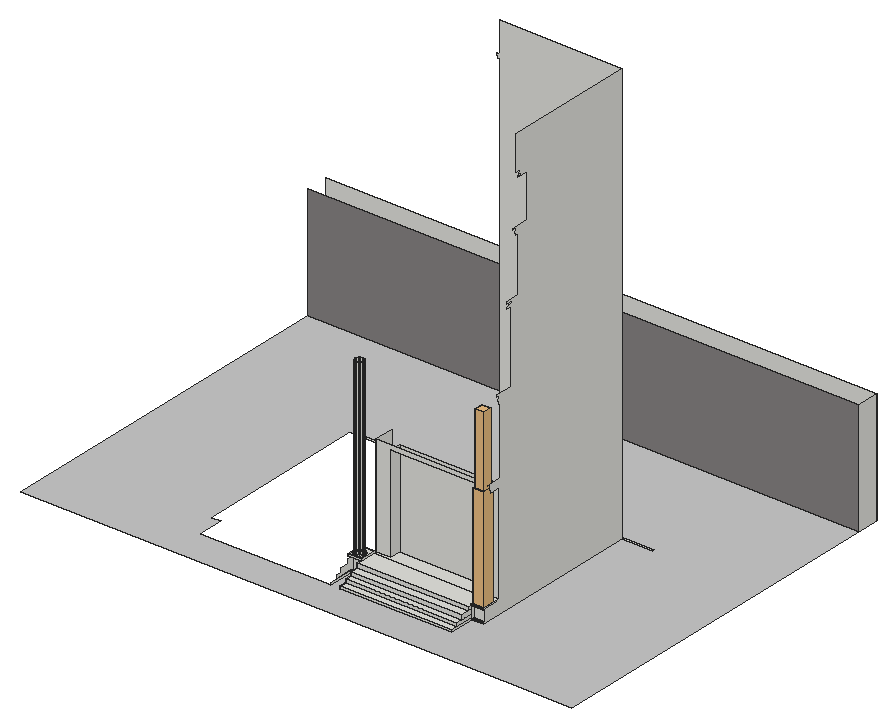
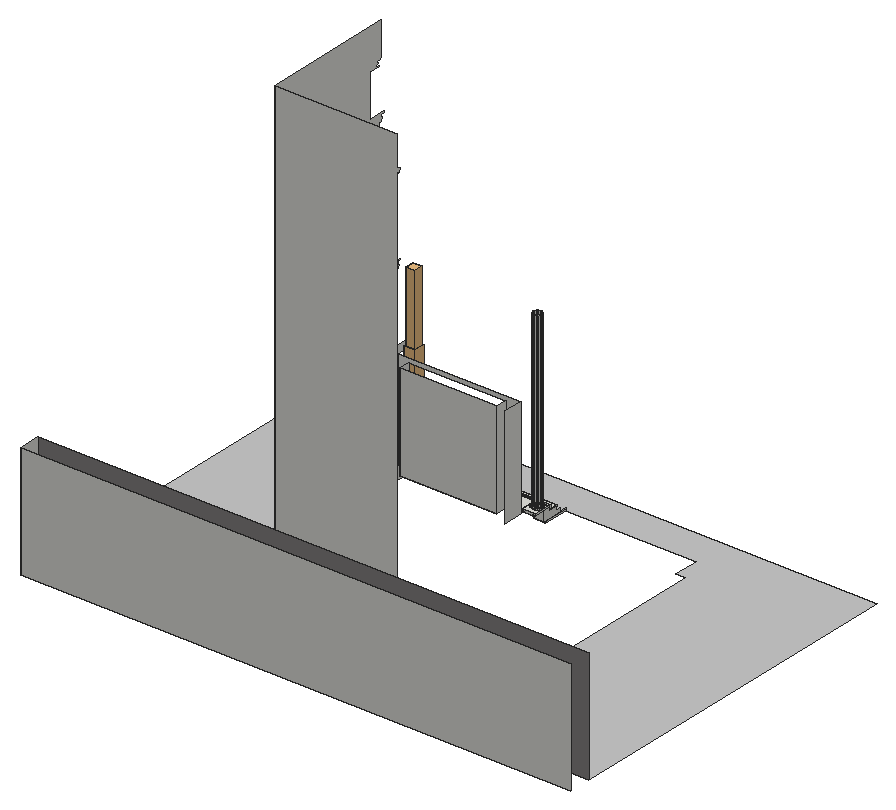
# SketchUp Ruby script. Lengths in inches.
U = 1.inch
M = Sketchup.active_model
def pt(a) = Geom::Point3d.new(a.map { |v| v * U })
def face(e, loops, mat)
  f = e.add_face(loops[0].map { |a| pt(a) })
  loops[1..].each { |l| e.add_face(l.map { |a| pt(a) }).erase! }
  f.material = f.back_material = mat if mat
  f
end
# faces: each face lists its corners as indices into pts; further lists are holes
def faces(e, pts, list, mat = nil) = list.each { |f| face(e, (f[0].is_a?(Array) ? f : [f]).map { |l| l.map { |i| pts[i] } }, mat) }
# xy, xz, yz: faces in a plane at the given z, y or x. An outline is a flat list of corners, or four numbers for a rectangle; further outlines are holes
def ring(l) = l.size == 4 ? [[l[0], l[1]], [l[2], l[1]], [l[2], l[3]], [l[0], l[3]]] : l.each_slice(2).to_a
def flat(e, list, mat, &to3) = list.each { |f| face(e, (f[0].is_a?(Array) ? f : [f]).map { |l| ring(l).map { |u, v| to3.(u, v) } }, mat) }
def xy(e, z, list, mat = nil) = flat(e, list, mat) { |x, y| [x, y, z] }
def xz(e, y, list, mat = nil) = flat(e, list, mat) { |x, z| [x, y, z] }
def yz(e, x, list, mat = nil) = flat(e, list, mat) { |y, z| [x, y, z] }
def lines(e, pts, list) = list.each { |a, b| e.add_line(pt(pts[a]), pt(pts[b])) }
# prism: a flat outline (further loops are holes) pulled along v
def prism(e, loops, v, mat = nil)
  f = face(e, loops, mat); d = Geom::Vector3d.new(v.map { |x| x * U })
  f.pushpull(f.normal.samedirection?(d) ? d.length : -d.length)
end
def box(e, o, s, mat = nil) = prism(e, [[o, [o[0] + s[0], o[1], o[2]], [o[0] + s[0], o[1] + s[1], o[2]], [o[0], o[1] + s[1], o[2]]]], [0, 0, s[2]], mat)
def at(x, y, z, deg = 0) = Geom::Transformation.translation(pt([x, y, z])) * Geom::Transformation.rotation(ORIGIN, Z_AXIS, deg.degrees)
def axes(o, x, y, z) = Geom::Transformation.new([*x, 0, *y, 0, *z, 0, *pt(o).to_a, 1])
def part(name) = M.definitions.add(name)
# library, detail: a bought-in or finely detailed component or shape, given as its bounding box
def library(name, o, s) = part(name).tap { |d| box(d.entities, o, s) }
def detail(e, o, s) = box(e.add_group.entities, o, s)
def put(e, d, t, mat = nil) = e.add_instance(d, t).tap { |i| i.material = mat if mat }
def group(e, t, mat = nil) = e.add_group.tap { |g| g.transformation = t; g.material = mat if mat }.entities
root = M.entities
M.materials.add("[Brick Tumbled]").color = [135, 132, 132]
M.materials.add("[Cladding Stucco White]").color = [200, 200, 200]
c1 = library("Group\#1",[0,0,0],[8.125,8.125,76.3125])
xy(root,0,[[107.37,172.5625,326.68,174.07],[326.68,264.36,404.87,280.51]])
xy(root,0,[[0,0,355.49,0,355.49,0.34,404.87,0.34,404.87,264.36,326.68,264.36,326.68,172.5625,304.48,172.5625,304.48,44.88,295.89,44.88,295.89,26.25,214.17,26.25,214.17,44.88,207.4,44.88,207.4,26.25,111.24,26.25,111.24,44.88,104.23,44.88,104.23,172.5625,107.37,172.5625,107.37,174.07,326.68,174.07,326.68,264.36,0,264.36]],"[Cladding Stucco White]")
xy(root,0.71,[[296.3,44.88,304.48,45.25]])
xy(root,0.92,[[296.3,45.25,304.48,46.63]])
xy(root,1.01,[[207.37,26.25,207.4,44.88],[207.4,44.88,214.17,45.32]])
xy(root,1.55,[[207.37,45.32,214.17,46.63]])
xy(root,3.94,[[214.17,31.63,295.89,35.75]])
xy(root,6.875,[[214.17,35.75,295.89,41.88]])
xy(root,9.8125,[[214.17,41.88,295.89,41.88,295.89,56.16,214.17,56.57],[295.89,44.44,295.89,44.88,296.3,44.88,296.3,46.63,304.48,46.63,304.48,44.88,304.66,44.88,304.66,44.44],[304.48,44.88,304.66,56.12],[295.89,56.16,296.02,56.16,296.02,57.2,296.52,57.2,296.52,67.33,225.14,67.33,225.14,59.39,214.17,59.39,214.17,56.57]])
xy(root,10.4375,[[[295.89,44.44,304.66,44.44,304.66,56.12,304.48,56.12,304.48,59.39,296.52,59.39,296.52,57.2,296.02,57.2,296.02,56.16,295.89,56.16],[300.02,45.77,298.97,45.93,298,46.36,297.17,47.02,296.54,47.87,296.15,48.86,296.03,49.91,296.19,50.96,296.62,51.93,297.28,52.76,298.13,53.39,299.12,53.78,300.18,53.9,301.22,53.74,302.2,53.3125,303.02,52.65,303.65,51.8,304.04,50.81,304.16,49.75,304,48.71,303.57,47.73,302.91,46.91,302.06,46.28,301.07,45.89]]])
xy(root,10.75,[[205.39,44.25,205.39,44.88,206.95,44.88,206.95,46.44,207.18,46.125,208.01,45.46,208.98,45.04,210.03,44.88,211.08,45,212.07,45.38,212.93,46.01,213.42,46.63,214.17,46.63,214.17,44.88,215.3,44.88,215.3,44.25],[205.39,44.88,205.39,47.4,206.39,47.4,206.55,46.98,206.95,46.44,206.95,44.88],[210.03,44.88,208.98,45.04,208.01,45.46,207.18,46.125,206.95,46.44,206.95,46.63,210.03,46.63],[210.03,44.88,210.03,46.63,213.42,46.63,212.93,46.01,212.07,45.38,211.08,45],[214.17,44.88,215.3,56.57],
  [206.95,46.44,206.55,46.98,206.39,47.4,205.39,47.4,205.39,50.48,206.39,50.48,206.63,51.04,206.95,51.4375],[205.39,50.48,205.39,56.57,206.95,56.57,206.95,51.4375,206.63,51.04,206.39,50.48]])
xy(root,11.6875,[[205.39,44.25,215.3,56.57]])
xy(root,12,[[[210.03,44.88,211.08,45,212.07,45.38,212.93,46.01,213.59,46.84,214.01,47.8125,214.17,48.86,214.05,49.91,213.67,50.9,213.04,51.76,212.21,52.42,211.24,52.84,210.19,53,209.14,52.89,208.15,52.5,207.29,51.87,206.63,51.04,206.21,50.07,206.05,49.02,206.17,47.97,206.55,46.98,207.18,46.125,208.01,45.46,208.98,45.04],[210.04,45.32,209.1,45.46,208.23,45.84,207.5,46.43,206.93,47.19,206.59,48.07,206.48,49.01,206.625,49.95,207.01,50.82,207.6,51.56,208.36,52.12,209.24,52.46,210.18,52.57,211.12,52.43,211.98,52.05,212.72,51.45,213.29,50.69,213.63,49.81,213.74,48.87,213.59,47.93,213.21,47.07,212.62,46.33,211.86,45.77,210.98,45.42]]])
xy(root,12.875,[[[210.04,45.32,210.98,45.42,211.86,45.77,212.62,46.33,213.21,47.07,213.59,47.93,213.74,48.87,213.63,49.81,213.29,50.69,212.72,51.45,211.98,52.05,211.12,52.43,210.18,52.57,209.24,52.46,208.36,52.12,207.6,51.56,207.01,50.82,206.625,49.95,206.48,49.01,206.59,48.07,206.93,47.19,207.5,46.43,208.23,45.84,209.1,45.46],[210.05,45.88,209.26,46,208.53,46.32,207.9,46.82,207.43,47.46,207.14,48.21,207.05,49,207.17,49.79,207.49,50.52,207.99,51.15,208.63,51.625,209.375,51.91,210.17,52,210.96,51.88,211.69,51.5625,212.32,51.0625,212.79,50.42,213.08,49.68,213.17,48.88,213.05,48.09,212.73,47.36,212.23,46.73,211.59,46.26,210.84,45.97]]])
xy(root,15.4375,[[[210.09,45.77,210.9,45.86,211.66,46.15,212.32,46.63,212.83,47.27,213.15,48.02,213.28,48.83,213.1875,49.64,212.89,50.4,212.41,51.06,211.77,51.57,211.02,51.89,210.22,52.02,209.41,51.93,208.65,51.63,207.99,51.15,207.48,50.51,207.15,49.77,207.03,48.96,207.11,48.15,207.41,47.39,207.89,46.73,208.53,46.22,209.28,45.89],[210.05,46.14,209.33,46.25,208.66,46.55,208.09,47,207.66,47.59,207.39,48.27,207.3125,49,207.42,49.72,207.72,50.39,208.17,50.96,208.76,51.39,209.44,51.66,210.17,51.74,210.89,51.63,211.56,51.34,212.125,50.88,212.56,50.29,212.83,49.61,212.91,48.89,212.8,48.16,212.5,47.5,212.05,46.92,211.46,46.49,210.78,46.23]]])
xy(root,15.5625,[[[210.05,45.68,210.89,45.77,211.6875,46.08,212.37,46.59,212.9,47.25,213.25,48.03,213.375,48.875,213.28,49.72,212.97,50.52,212.46,51.2,211.8,51.74,211.02,52.08,210.17,52.21,209.33,52.11,208.53,51.8,207.85,51.3,207.32,50.63,206.97,49.85,206.85,49.01,206.94,48.16,207.25,47.37,207.76,46.68,208.42,46.15,209.2,45.81],[210.09,45.77,209.28,45.89,208.53,46.22,207.89,46.73,207.41,47.39,207.11,48.15,207.03,48.96,207.15,49.77,207.48,50.51,207.99,51.15,208.65,51.63,209.41,51.93,210.22,52.02,211.02,51.89,211.77,51.57,212.41,51.06,212.89,50.4,213.1875,49.64,213.28,48.83,213.15,48.02,212.83,47.27,212.32,46.63,211.66,46.15,210.9,45.86]]])
xz(root,26.25,[[214.17,0,295.89,0,295.89,1.36,214.17,1.55]])
xz(root,31.63,[[295.89,1.36,295.89,3.94,214.17,3.94,214.17,1.55]])
xz(root,35.75,[[214.17,3.94,295.89,6.875]])
xz(root,41.88,[[214.17,6.875,295.89,9.8125]])
xz(root,44.25,[[205.39,10.75,215.3,11.6875]])
xz(root,44.44,[[295.89,9.8125,304.66,10.4375]])
xz(root,44.88,[[207.4,0,207.45,0,207.4,1.01],[207.45,0,214.17,0,214.17,1.01,207.4,1.01],[295.89,0,296.3,0,296.3,1.35,295.89,1.36],[296.3,0,304.48,0.71],[207.37,1.01,207.4,1.01,207.37,1.55],
  [296.3,1.35,296.3,9.8125,295.89,9.8125,295.89,1.36]])
xz(root,45.25,[[296.3,0.71,304.48,0.92]])
xz(root,45.32,[[207.4,1.01,214.17,1.01,214.17,1.55,207.37,1.55]])
xz(root,46.63,[[296.3,0.92,304.48,9.8125],[207.37,1.55,214.17,1.55,214.17,10.75,206.95,10.75,206.95,9.8125]])
xz(root,56.12,[[304.48,9.8125,304.66,10.4375]])
xz(root,56.16,[[295.89,9.8125,296.02,10.4375]])
xz(root,56.57,[[206.95,9.8125,206.95,10.75,205.39,10.75,205.39,11.6875,215.3,11.6875,215.3,10.75,214.17,10.75,214.17,9.8125]])
xz(root,57.2,[[296.02,9.8125,296.52,10.4375]])
xz(root,59.39,[[214.17,9.8125,225.14,9.8125,225.14,80.55,296.52,80.55,296.52,10.4375,304.48,10.4375,304.48,83.64,214.17,83.64]])
xz(root,67.33,[[225.14,9.8125,296.52,80.55]])
xz(root,172.5625,[[214.17,0,214.17,284.98,212.73,284.98,212.73,286.66,212.55,286.66,212.55,288.01,214.17,288.01,214.17,309.9375,304.48,309.9375,304.48,0]])
xz(root,264.36,[[0,0,404.87,83.4375]],"[Brick Tumbled]")
xz(root,280.51,[[0,0,404.87,83.4375]])
yz(root,205.39,[[44.25,10.75,56.57,11.6875]])
yz(root,206.95,[[46.63,9.8125,56.57,10.75]])
yz(root,207.37,[[26.25,1.01,44.88,1.55]])
yz(root,207.4,[[26.25,0,44.88,1.01]])
yz(root,214.17,[[26.25,0,44.88,1.01],[26.25,1.01,45.32,1.55],[31.63,1.55,31.63,3.94,35.75,3.94,35.75,6.875,41.88,6.875,41.88,9.8125,46.63,9.8125,46.63,1.55],[46.63,9.8125,56.57,10.75],[59.39,9.8125,73.64,83.92]])
yz(root,215.3,[[44.25,10.75,56.57,11.6875]])
yz(root,225.14,[[59.39,9.8125,67.33,80.55]])
yz(root,295.89,[[26.25,0,44.88,1.36],[31.63,1.36,44.88,3.94],[35.75,3.94,44.88,6.875],[41.88,6.875,44.88,9.8125],[44.44,9.8125,56.16,10.4375]])
yz(root,296.02,[[56.16,9.8125,57.2,10.4375]])
yz(root,296.3,[[44.88,0.71,45.25,1.35],[45.25,0.92,46.63,0.92,46.63,9.8125,44.88,9.8125,44.88,1.35,45.25,1.35]])
yz(root,296.52,[[57.2,9.8125,57.2,10.4375,59.39,10.4375,59.39,80.55,67.33,80.55,67.33,9.8125]])
yz(root,304.48,[[44.88,0,172.5625,0,172.5625,309.9375,74.52,309.9375,74.52,284.98,75.52,284.98,75.52,284.33,78.58,284.33,78.58,282.84,77.08,282.84,77.08,282.12,79.14,282.12,79.14,281.14,76.7,281.14,76.7,280.4,85.02,280.4,85.02,248.6875,71.75,248.6875,71.75,247.95,74.625,247.95,74.625,245.88,73.625,245.88,73.625,244.86,74.375,244.86,74.375,243.8,75.125,243.8,75.125,243.18,76.3125,243.18,76.3125,202.875,66.1875,202.875,66.1875,201.42,71,201.42,71,199.99,68.5625,199.99,68.5625,199.04,66.56,199.04,66.56,197.93,70.1875,197.93,70.1875,145.3125,57.25,145.3125,57.25,144.42,59.19,144.42,59.19,141.75,58,141.75,58,141.14,59.06,141.14,59.06,139.125,60.44,139.125,60.44,89.5625,49.08,89.5625,49.08,89.28,50.51,89.28,50.51,86.32,51.58,86.32,51.58,83.64,59.39,83.64,59.39,10.4375,56.12,10.4375,56.12,9.8125,46.63,9.8125,46.63,0.92,45.25,0.92,45.25,0.71,44.88,0.71]])
yz(root,304.66,[[44.44,9.8125,56.12,10.4375]])
yz(root,404.87,[[264.36,0,280.51,83.4375]])
p = [[207.37,44.88,1.55],[207.4,44.88,1.01],[207.4,45.32,1.01],[207.37,45.32,1.55],[295.89,26.25,1.36],[295.89,31.63,1.36],
  [214.17,31.63,1.55],[214.17,26.25,1.55],[206.95,46.63,9.8125],[206.95,41.88,9.8125],[207.1,41.88,6.88],[207.1,35.75,6.88],
  [207.25,35.75,3.95],[207.25,31.63,3.95],[207.37,31.63,1.55],[207.37,46.63,1.55],[213.42,46.63,10.75],[213.59,46.84,10.75],
  [213.59,46.84,12],[212.93,46.01,12],[212.93,46.01,10.75],[206.95,46.44,10.75],[207.18,46.125,10.75],[207.18,46.125,12],
  [206.55,46.98,12],[206.55,46.98,10.75],[214.01,47.8125,10.75],[214.01,47.8125,12],[206.39,47.4,10.75],[206.17,47.97,12],
  [206.17,47.97,10.75],[214.17,48.86,10.75],[214.17,48.86,12],[206.05,49.02,10.75],[206.05,49.02,12],[214.05,49.91,10.75],
  [214.05,49.91,12],[206.21,50.07,10.75],[206.21,50.07,12],[213.67,50.9,10.75],[213.67,50.9,12],[206.39,50.48,10.75],
  [206.63,51.04,12],[206.63,51.04,10.75],[213.04,51.76,10.75],[213.04,51.76,12],[206.95,51.4375,10.75],[207.29,51.87,12],
  [207.29,51.87,10.75],[212.21,52.42,10.75],[212.21,52.42,12],[208.15,52.5,10.75],[208.15,52.5,12],[211.24,52.84,10.75],
  [211.24,52.84,12],[209.14,52.89,10.75],[209.14,52.89,12],[210.19,53,10.75],[210.19,53,12],[208.98,45.04,10.75],
  [210.03,44.88,10.75],[210.03,44.88,12],[208.98,45.04,12],[211.08,45,10.75],[211.08,45,12],[208.01,45.46,10.75],
  [208.01,45.46,12],[212.07,45.38,10.75],[212.07,45.38,12],[209.1,45.46,12],[210.04,45.32,12],[210.04,45.32,12.875],
  [209.1,45.46,12.875],[210.98,45.42,12],[210.98,45.42,12.875],[211.86,45.77,12],[211.86,45.77,12.875],[208.23,45.84,12],
  [208.23,45.84,12.875],[207.5,46.43,12],[207.5,46.43,12.875],[212.62,46.33,12],[212.62,46.33,12.875],[213.21,47.07,12],
  [213.21,47.07,12.875],[206.93,47.19,12],[206.93,47.19,12.875],[213.59,47.93,12],[213.59,47.93,12.875],[206.59,48.07,12],
  [206.59,48.07,12.875],[213.74,48.87,12],[213.74,48.87,12.875],[206.48,49.01,12],[206.48,49.01,12.875],[213.63,49.81,12],
  [213.63,49.81,12.875],[206.625,49.95,12],[206.625,49.95,12.875],[213.29,50.69,12],[213.29,50.69,12.875],[207.01,50.82,12],
  [207.01,50.82,12.875],[212.72,51.45,12],[212.72,51.45,12.875],[207.6,51.56,12],[207.6,51.56,12.875],[211.98,52.05,12],
  [211.98,52.05,12.875],[208.36,52.12,12],[208.36,52.12,12.875],[211.12,52.43,12],[211.12,52.43,12.875],[209.24,52.46,12],
  [209.24,52.46,12.875],[210.18,52.57,12],[210.18,52.57,12.875],[210.05,45.88,139.125],[209.26,46,139.125],[209.26,46,12.875],
  [210.05,45.88,12.875],[210.84,45.97,139.125],[210.84,45.97,12.875],[208.53,46.32,139.125],[208.53,46.32,12.875],[211.59,46.26,139.125],
  [211.59,46.26,12.875],[207.9,46.82,139.125],[207.9,46.82,12.875],[212.23,46.73,139.125],[212.23,46.73,12.875],[212.73,47.36,139.125],
  [212.73,47.36,12.875],[207.43,47.46,139.125],[207.43,47.46,12.875],[213.05,48.09,139.125],[213.05,48.09,12.875],[207.14,48.21,139.125],
  [207.14,48.21,12.875],[213.17,48.88,139.125],[213.17,48.88,12.875],[207.05,49,139.125],[207.05,49,12.875],[213.08,49.68,139.125],
  [213.08,49.68,12.875],[207.17,49.79,139.125],[207.17,49.79,12.875],[212.79,50.42,139.125],[212.79,50.42,12.875],[207.49,50.52,139.125],
  [207.49,50.52,12.875],[212.32,51.0625,139.125],[212.32,51.0625,12.875],[207.99,51.15,139.125],[207.99,51.15,15.5625],[207.99,51.15,15.4375],
  [207.99,51.15,14.6875],[207.99,51.15,12.875],[208.63,51.625,139.125],[208.63,51.625,12.875],[211.69,51.5625,139.125],[211.69,51.5625,12.875],
  [209.375,51.91,139.125],[209.375,51.91,12.875],[210.96,51.88,139.125],[210.96,51.88,12.875],[210.17,52,139.125],[210.17,52,12.875],
  [209.28,45.89,14.6875],[210.09,45.77,14.6875],[210.09,45.77,15.4375],[209.28,45.89,15.4375],[210.9,45.86,14.6875],[210.9,45.86,15.4375],
  [208.53,46.22,14.6875],[208.53,46.22,15.4375],[211.66,46.15,14.6875],[211.66,46.15,15.4375],[207.89,46.73,14.6875],[207.89,46.73,15.4375],
  [212.32,46.63,14.6875],[212.32,46.63,15.4375],[212.83,47.27,14.6875],[212.83,47.27,15.4375],[207.41,47.39,14.6875],[207.41,47.39,15.4375],
  [213.15,48.02,14.6875],[213.15,48.02,15.4375],[207.11,48.15,14.6875],[207.11,48.15,15.4375],[213.28,48.83,14.6875],[213.28,48.83,15.4375],
  [207.03,48.96,14.6875],[207.03,48.96,15.4375],[213.1875,49.64,14.6875],[213.1875,49.64,15.4375],[207.15,49.77,14.6875],[207.15,49.77,15.4375],
  [212.89,50.4,14.6875],[212.89,50.4,15.4375],[207.48,50.51,14.6875],[207.48,50.51,15.4375],[212.41,51.06,14.6875],[212.41,51.06,15.4375],
  [208.65,51.63,14.6875],[208.65,51.63,15.4375],[211.77,51.57,14.6875],[211.77,51.57,15.4375],[209.41,51.93,14.6875],[209.41,51.93,15.4375],
  [211.02,51.89,14.6875],[211.02,51.89,15.4375],[210.22,52.02,14.6875],[210.22,52.02,15.4375],[209.2,45.81,15.4375],[210.05,45.68,15.4375],
  [210.05,45.68,15.5625],[209.2,45.81,15.5625],[210.89,45.77,15.4375],[210.89,45.77,15.5625],[208.42,46.15,15.4375],[208.42,46.15,15.5625],
  [209.28,45.89,15.5625],[210.09,45.77,15.5625],[210.9,45.86,15.5625],[211.6875,46.08,15.4375],[211.6875,46.08,15.5625],[208.53,46.22,15.5625],
  [211.66,46.15,15.5625],[207.76,46.68,15.4375],[207.76,46.68,15.5625],[212.37,46.59,15.4375],[212.37,46.59,15.5625],[207.89,46.73,15.5625],
  [212.32,46.63,15.5625],[212.83,47.27,15.5625],[212.9,47.25,15.4375],[212.9,47.25,15.5625],[207.25,47.37,15.4375],[207.25,47.37,15.5625],
  [207.41,47.39,15.5625],[213.15,48.02,15.5625],[213.25,48.03,15.4375],[213.25,48.03,15.5625],[206.94,48.16,15.4375],[206.94,48.16,15.5625],
  [207.11,48.15,15.5625],[213.28,48.83,15.5625],[213.375,48.875,15.4375],[213.375,48.875,15.5625],[207.03,48.96,15.5625],[206.85,49.01,15.4375],
  [206.85,49.01,15.5625],[213.1875,49.64,15.5625],[213.28,49.72,15.4375],[213.28,49.72,15.5625],[206.97,49.85,15.4375],[206.97,49.85,15.5625],
  [207.15,49.77,15.5625],[212.89,50.4,15.5625],[212.97,50.52,15.4375],[212.97,50.52,15.5625],[207.32,50.63,15.4375],[207.32,50.63,15.5625],
  [207.48,50.51,15.5625],[212.41,51.06,15.5625],[212.46,51.2,15.4375],[212.46,51.2,15.5625],[207.85,51.3,15.4375],[207.85,51.3,15.5625],
  [208.65,51.63,15.5625],[211.77,51.57,15.5625],[211.8,51.74,15.4375],[211.8,51.74,15.5625],[208.53,51.8,15.4375],[208.53,51.8,15.5625],
  [209.41,51.93,15.5625],[211.02,51.89,15.5625],[211.02,52.08,15.4375],[211.02,52.08,15.5625],[209.33,52.11,15.4375],[209.33,52.11,15.5625],
  [210.22,52.02,15.5625],[210.17,52.21,15.4375],[210.17,52.21,15.5625],[207.63,48.99,14.6875],[207.73,49.63,14.6875],[207.71,48.35,14.6875],
  [208.83,46.82,14.6875],[208.32,47.23,14.6875],[207.94,47.75,14.6875],[211.31,46.77,14.6875],[210.7,46.54,14.6875],[207.99,50.22,14.6875],
  [208.39,50.73,14.6875],[212.49,48.25,14.6875],[212.23,47.66,14.6875],[211.83,47.16,14.6875],[210.0625,46.47,14.6875],[208.91,51.11,14.6875],
  [209.52,51.35,14.6875],[212.59,48.89,14.6875],[212.51,49.53,14.6875],[209.42,46.5625,14.6875],[212.28,50.14,14.6875],[210.16,51.42,14.6875],
  [210.8,51.32,14.6875],[211.39,51.0625,14.6875],[211.89,50.66,14.6875]]
faces(root,p,[[0,1,2,3],[4,5,6,7],[8,9,10,11,12,13,14,0,3,15],[16,17,18,19,20],[21,22,23,24,25],[17,26,27,18],[28,25,24,29,30],[26,31,32,27],
  [33,30,29,34],[31,35,36,32],[37,33,34,38],[35,39,40,36],[41,37,38,42,43],[39,44,45,40],[46,43,42,47,48],[44,49,50,45],
  [51,48,47,52],[49,53,54,50],[55,51,52,56],[53,57,58,54],[57,55,56,58],[59,60,61,62],[60,63,64,61],[65,59,62,66],
  [63,67,68,64],[67,20,19,68],[22,65,66,23],[69,70,71,72],[70,73,74,71],[73,75,76,74],[77,69,72,78],[79,77,78,80],
  [75,81,82,76],[81,83,84,82],[85,79,80,86],[83,87,88,84],[89,85,86,90],[87,91,92,88],[93,89,90,94],[91,95,96,92],
  [97,93,94,98],[95,99,100,96],[101,97,98,102],[99,103,104,100],[105,101,102,106],[103,107,108,104],[109,105,106,110],[107,111,112,108],
  [113,109,110,114],[111,115,116,112],[115,113,114,116],[117,118,119,120],[121,117,120,122],[118,123,124,119],[125,121,122,126],[123,127,128,124],
  [129,125,126,130],[131,129,130,132],[127,133,134,128],[135,131,132,136],[133,137,138,134],[139,135,136,140],[137,141,142,138],[143,139,140,144],
  [141,145,146,142],[147,143,144,148],[145,149,150,146],[151,147,148,152],[149,153,154,155,156,157,150],[153,158,159,157,156,155,154],[160,151,152,161],[158,162,163,159],
  [164,160,161,165],[162,166,167,163],[166,164,165,167],[168,169,170,171],[169,172,173,170],[174,168,171,175],[172,176,177,173],[178,174,175,179],
  [176,180,181,177],[180,182,183,181],[184,178,179,185],[182,186,187,183],[188,184,185,189],[186,190,191,187],[192,188,189,193],[190,194,195,191],
  [196,192,193,197],[194,198,199,195],[200,196,197,201],[198,202,203,199],[156,200,201,155],[204,156,155,205],[202,206,207,203],[208,204,205,209],
  [206,210,211,207],[212,208,209,213],[210,212,213,211],[214,215,216,217],[215,218,219,216],[220,214,217,221],[170,171,222,223],[173,170,223,224],
  [218,225,226,219],[171,175,227,222],[177,173,224,228],[229,220,221,230],[225,231,232,226],[175,179,233,227],[181,177,228,234],[183,181,234,235],
  [231,236,237,232],[238,229,230,239],[179,185,240,233],[187,183,235,241],[236,242,243,237],[244,238,239,245],[185,189,246,240],[191,187,241,247],
  [242,248,249,243],[189,193,250,246],[251,244,245,252],[195,191,247,253],[248,254,255,249],[256,251,252,257],[193,197,258,250],[199,195,253,259],
  [254,260,261,255],[262,256,257,263],[197,201,264,258],[203,199,259,265],[201,155,154,264],[260,266,267,261],[268,262,263,269],[155,205,270,154],
  [207,203,265,271],[266,272,273,267],[274,268,269,275],[205,209,276,270],[211,207,271,277],[272,278,279,273],[280,274,275,281],[209,213,282,276],
  [213,211,277,282],[283,280,281,284],[278,283,284,279]])
lines(root,p,[[285,286],[287,285],[288,289],[289,290],[291,292],[293,294],[290,287],[295,296],[297,291],[292,298],[299,300],[294,299],
  [296,297],[301,295],[302,301],[298,303],[304,302],[286,293],[303,288],[305,306],[307,308],[300,305],[308,304],[306,307]])
detail(root,[296.83,46.57,14.375],[6.53,6.53,124.0625])
put(root,c1,at(296.03,45.77,10.4375))
